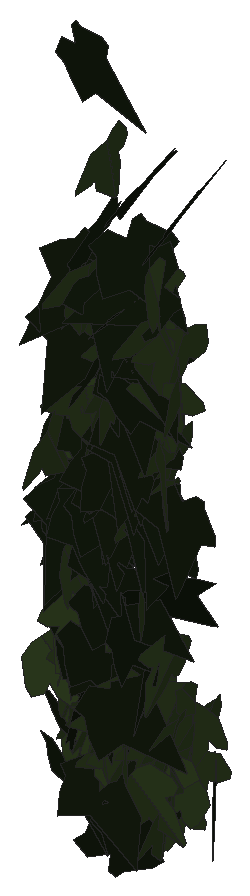
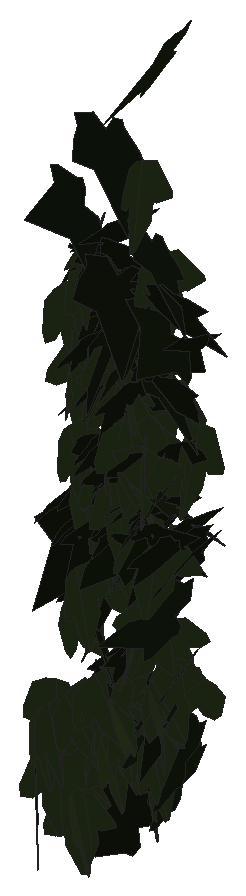
# SketchUp Ruby script. Lengths in inches.
U = 1.inch
M = Sketchup.active_model
def pt(a) = Geom::Point3d.new(a.map { |v| v * U })
def face(e, loops, mat)
  f = e.add_face(loops[0].map { |a| pt(a) })
  loops[1..].each { |l| e.add_face(l.map { |a| pt(a) }).erase! }
  f.material = f.back_material = mat if mat
  f
end
# faces: each face lists its corners as indices into pts; further lists are holes
def faces(e, pts, list, mat = nil) = list.each { |f| face(e, (f[0].is_a?(Array) ? f : [f]).map { |l| l.map { |i| pts[i] } }, mat) }
# xy, xz, yz: faces in a plane at the given z, y or x. An outline is a flat list of corners, or four numbers for a rectangle; further outlines are holes
def ring(l) = l.size == 4 ? [[l[0], l[1]], [l[2], l[1]], [l[2], l[3]], [l[0], l[3]]] : l.each_slice(2).to_a
def flat(e, list, mat, &to3) = list.each { |f| face(e, (f[0].is_a?(Array) ? f : [f]).map { |l| ring(l).map { |u, v| to3.(u, v) } }, mat) }
def xy(e, z, list, mat = nil) = flat(e, list, mat) { |x, y| [x, y, z] }
def xz(e, y, list, mat = nil) = flat(e, list, mat) { |x, z| [x, y, z] }
def yz(e, x, list, mat = nil) = flat(e, list, mat) { |y, z| [x, y, z] }
def lines(e, pts, list) = list.each { |a, b| e.add_line(pt(pts[a]), pt(pts[b])) }
# prism: a flat outline (further loops are holes) pulled along v
def prism(e, loops, v, mat = nil)
  f = face(e, loops, mat); d = Geom::Vector3d.new(v.map { |x| x * U })
  f.pushpull(f.normal.samedirection?(d) ? d.length : -d.length)
end
def box(e, o, s, mat = nil) = prism(e, [[o, [o[0] + s[0], o[1], o[2]], [o[0] + s[0], o[1] + s[1], o[2]], [o[0], o[1] + s[1], o[2]]]], [0, 0, s[2]], mat)
def at(x, y, z, deg = 0) = Geom::Transformation.translation(pt([x, y, z])) * Geom::Transformation.rotation(ORIGIN, Z_AXIS, deg.degrees)
def axes(o, x, y, z) = Geom::Transformation.new([*x, 0, *y, 0, *z, 0, *pt(o).to_a, 1])
def part(name) = M.definitions.add(name)
# library, detail: a bought-in or finely detailed component or shape, given as its bounding box
def library(name, o, s) = part(name).tap { |d| box(d.entities, o, s) }
def detail(e, o, s) = box(e.add_group.entities, o, s)
def put(e, d, t, mat = nil) = e.add_instance(d, t).tap { |i| i.material = mat if mat }
def group(e, t, mat = nil) = e.add_group.tap { |g| g.transformation = t; g.material = mat if mat }.entities
root = M.entities
M.materials.add("efeu1").color = [18, 25, 13]
M.materials.add("efeu2").color = [43, 57, 29]
c1 = part("ivyleaf_9")
p = [[1.54,2.16,1.25],[1.36,2.04,1.19],[-0.21,0.99,0.68],[-0.71,1.11,0.82],[-0.85,0.86,0.67],[-0.8,0.17,0.21],
  [-0.9,-0.01,0.1],[-0.67,-0.16,-0.02],[-0.08,-0.08,-0.05],[-0.03,-0.6,-0.4],[0.65,-0.88,-0.66],[0.83,-0.6,-0.49],
  [1.29,-0.42,-0.43],[1.8125,-0.07,-0.26],[1.21,0.44,0.15]]
faces(c1.entities,p,[[0,1,2,3,4,5,6,7,8,9,10,11,12,13,14]],"efeu1")
c2 = part("ivyleaf_10")
p = [[0,0.5,-0.03],[-0.0625,2.02,-0.43],[-0.19,2.01,-0.46],[-0.54,1.05,-0.29],[-0.52,0.625,-0.18],[-0.83,0.76,-0.28],
  [-1.16,0.64,-0.33],[-1.15,0.33,-0.24],[-0.77,-0.39,0.02],[-0.3,-0.51,0.16],[0.04,-0.48,0.23],[-0.02,2.01,-0.4375],
  [-0.06,2.01,-0.43],[0.04,-0.49,0.23],[0.67,-0.49,0.14],[1.38,0.36,-0.2],[1.375,0.51,-0.24],[0.81,0.65,-0.19],
  [0.62,0.59,-0.15],[0.6,1.09,-0.28],[0.5,1.23,-0.31]]
faces(c2.entities,p,[[0,1,2,3,4,5,6,7,8,9,10],[11,12,0,13,14,15,16,17,18,19,20]],"efeu2")
put(root,c1,axes([519.4,136.41,189.33],[0.62786,-0.42053,0.09806],[0.1674,0.07754,-0.73935],[0.39804,0.63072,0.15627]))
put(root,c2,axes([519.98,134.74,192.76],[0.04873,-0.68093,-0.48319],[0.02855,0.48508,-0.68073],[0.83446,0.02316,0.05151]))
put(root,c1,axes([519.65,136.01,190.9],[0.17877,-0.60551,-0.44438],[-0.02732,0.45125,-0.62586],[0.75058,0.16064,0.08305]))
put(root,c2,axes([519.98,136.06,187.02],[-0.04019,-0.69972,0.37768],[0.10675,-0.37948,-0.69171],[0.78794,0.01572,0.11298]))
put(root,c2,axes([520.09,136.15,185.5],[0.02126,-0.75748,0.0329],[-0.00474,-0.03305,-0.75775],[0.75818,0.02103,-0.00566]))
put(root,c1,axes([519.84,135.76,189.91],[-0.09217,-0.66346,0.40385],[-0.01785,-0.40476,-0.66905],[0.77651,-0.08806,0.03256]))
put(root,c1,axes([520.24,135.45,195.7],[0.19526,0.4822,0.58386],[-0.07597,0.61239,-0.48036],[-0.75342,0.06322,0.19976]))
put(root,c2,axes([519.59,135.28,187.0625],[0.53061,0.2169,0.52994],[0.49579,0.18745,-0.57313],[-0.28649,0.72612,-0.01034]))
put(root,c2,axes([520.15,136.03,190.54],[-0.6067,-0.44748,-0.06254],[0.0541,0.03201,-0.75384],[0.44858,-0.60907,0.00633]))
put(root,c1,axes([519.57,135.82,185.35],[0.53841,-0.59019,0.23254],[0.1518,-0.17626,-0.79886],[0.61592,0.55937,-0.00638]))
put(root,c1,axes([520.35,136.34,190.97],[-0.6514,-0.3842,0.08037],[-0.05254,-0.06898,-0.75556],[0.38898,-0.6527,0.03254]))
put(root,c2,axes([520.12,135.96,186.95],[0.28744,-0.67212,0.24553],[0.10655,-0.22145,-0.73093],[0.70758,0.30638,0.01032]))
put(root,c1,axes([520.51,135.22,186.4],[-0.1296,0.18302,-0.8633],[-0.7072,0.50041,0.21225],[0.52789,0.71532,0.0724]))
put(root,c1,axes([520.49,135.65,196.62],[-0.76491,-0.15378,0.03302],[-0.03296,-0.00358,-0.78021],[0.15379,-0.76562,-0.00298]))
put(root,c1,axes([519.79,136.01,187.22],[0.46827,-0.69757,-0.12739],[-0.04858,0.12074,-0.83974],[0.70744,0.47002,0.02666]))
put(root,c2,axes([520.1,136.32,188.6875],[-0.70161,0.1002,-0.25745],[0.22922,-0.18107,-0.69516],[-0.1542,-0.72509,0.13802]))
put(root,c2,axes([520.3,135.5625,188.23],[0.64412,0.32436,-0.21371],[-0.20684,-0.06387,-0.72035],[-0.32878,0.67563,0.0345]))
put(root,c1,axes([520.16,135.81,190.6],[-0.24349,-0.77579,0.29791],[-0.04142,-0.29871,-0.81175],[0.82999,-0.2425,0.04688]))
put(root,c1,axes([520.25,135.73,195.21],[-0.32979,-0.68595,0.20589],[-0.04139,-0.20803,-0.7594],[0.71499,-0.32844,0.05101]))
put(root,c1,axes([519.98,136.4,191.83],[0.35759,-0.6709,0.03227],[0.01369,-0.02927,-0.76025],[0.67154,0.35785,-0.00169]))
put(root,c2,axes([520.42,135.93,192.8],[0.2286,-0.6462,-0.38629],[-0.02349,0.39738,-0.67866],[0.75249,0.20872,0.09616]))
put(root,c1,axes([520.81,135.3,197.67],[-0.37796,0.6646,0.18343],[-0.08653,0.16181,-0.76455],[-0.684,-0.38771,-0.00465]))
put(root,c1,axes([520.84,135.58,191.73],[-0.71734,0.25796,-0.01039],[-0.06316,-0.20511,-0.73155],[-0.25032,-0.68747,0.21436]))
put(root,c1,axes([520.2,136.01,192.9],[-0.15486,-0.71167,-0.27805],[0.12148,0.25716,-0.72586],[0.75433,-0.18751,0.05981]))
put(root,c1,axes([520.84,135.32,194.71],[-0.51151,0.57612,0.00569],[-0.0038,0.00424,-0.77043],[-0.57614,-0.51152,0.00003]))
put(root,c1,axes([519.96,135.39,184.47],[0.43787,-0.63856,0.29211],[0.15808,-0.24577,-0.77422],[0.68417,0.46546,-0.00807]))
put(root,c2,axes([520.54,135.58,185.8],[0.29672,-0.6997,-0.07179],[-0.03319,0.0639,-0.76],[0.70259,0.29852,-0.00558]))
put(root,c2,axes([520.61,135.62,186.35],[0.51304,-0.43163,-0.3141],[-0.17742,0.27302,-0.66495],[0.50347,0.53604,0.08575]))
put(root,c2,axes([520.17,136.1,192.6875],[0.56352,0.40652,0.34786],[0.27327,0.21566,-0.69472],[-0.45999,0.62614,0.01343]))
put(root,c1,axes([520.16,135.89,194.82],[-0.27577,-0.37786,-0.6264],[0.57469,0.30231,-0.43537],[0.45264,-0.61404,0.17112]))
put(root,c2,axes([520.66,134.69,189.99],[-0.13696,0.64036,0.37512],[-0.2095,0.33258,-0.64423],[-0.71196,-0.22105,0.11741]))
put(root,c1,axes([520.16,136.125,185.95],[0.17917,-0.60388,0.43948],[0.20261,-0.3957,-0.62633],[0.71886,0.26204,0.067]))
put(root,c2,axes([520.75,136.17,193.22],[-0.45908,-0.60779,0.09787],[-0.00657,-0.11724,-0.75891],[0.61558,-0.45452,0.06489]))
put(root,c2,axes([520.6,135.9,188.55],[0.35102,-0.52158,-0.4512],[0.08319,0.53461,-0.55328],[0.68462,0.20246,0.29857]))
put(root,c2,axes([520.68,135.84,199.6],[0.02593,-0.73809,-0.27683],[0.06451,0.27803,-0.73526],[0.78565,0.00153,0.06951]))
put(root,c2,axes([520.76,135.07,196.86],[-0.14423,-0.79271,-0.04404],[0.00998,0.04295,-0.80573],[0.79387,-0.14456,0.00213]))
put(root,c2,axes([520.59,136.78,186.67],[0.36325,-0.59799,0.30121],[0.14821,-0.26237,-0.69962],[0.65296,0.39223,-0.00877]))
put(root,c2,axes([520.6875,135.68,191.68],[0.40284,-0.70378,0.09839],[0.03079,-0.09571,-0.81065],[0.70996,0.40348,-0.02067]))
put(root,c1,axes([520.4,136.375,194.78],[0.21017,-0.66144,-0.31804],[-0.04099,0.31973,-0.69204],[0.73278,0.20759,0.05251]))
put(root,c2,axes([520.78,135.13,193.83],[-0.7091,-0.36715,-0.06502],[0.0577,0.02998,-0.79851],[0.36837,-0.71145,-0.00009]))
put(root,c2,axes([520.78,135.5,184.5],[0.45996,-0.53802,-0.18395],[-0.06451,0.1857,-0.70443],[0.56493,0.45925,0.06933]))
put(root,c2,axes([520.36,135.32,185.7],[0.43547,-0.05792,0.65914],[0.64967,-0.11225,-0.43908],[0.12551,0.78199,-0.01421]))
put(root,c1,axes([520.58,135.03,202.44],[0.60057,-0.47896,-0.30462],[-0.14232,0.30225,-0.75583],[0.54949,0.60177,0.13718]))
put(root,c2,axes([521.03,136.11,191.62],[-0.30817,-0.70176,-0.06135],[0.02405,0.05644,-0.76644],[0.70402,-0.30911,-0.00067]))
put(root,c1,axes([520.73,135.34,190.98],[0.00331,-0.75327,-0.10452],[0.00542,0.10454,-0.75325],[0.76047,0.00254,0.00582]))
put(root,c2,axes([521.02,135.62,194.07],[0.23431,-0.72389,0.15536],[0.03955,-0.15048,-0.76082],[0.73932,0.23747,-0.00854]))
put(root,c2,axes([520.53,135.98,193.67],[0.56017,-0.01498,0.54702],[0.54381,0.10249,-0.55408],[-0.061,0.77621,0.08372]))
put(root,c1,axes([520.63,136.2,190.86],[0.72569,-0.23795,-0.02613],[-0.02865,-0.00352,-0.76361],[0.23766,0.72615,-0.01227]))
put(root,c1,axes([521.29,135.93,196.92],[-0.04492,0.78645,0.02013],[-0.00595,0.01982,-0.78771],[-0.78668,-0.04506,0.00481]))
put(root,c1,axes([520.83,135.42,187.8],[0.18152,-0.58271,-0.50064],[-0.12002,0.48659,-0.60988],[0.7588,0.21636,0.02329]))
put(root,c1,axes([521,135.99,190.78],[-0.23052,-0.72721,0.07545],[-0.03857,-0.0669,-0.7627],[0.7301,-0.23314,-0.01647]))
put(root,c2,axes([521.23,135.86,194.88],[-0.55356,-0.56218,-0.01701],[0.01551,0.0086,-0.78895],[0.56222,-0.55375,0.00502]))
put(root,c1,axes([520.86,135.32,191.36],[0.32309,-0.53201,-0.48751],[-0.13922,0.47815,-0.61406],[0.70803,0.33678,0.10171]))
put(root,c1,axes([521,135.81,192.03],[-0.17758,-0.73878,-0.07039],[0.00817,0.07043,-0.75977],[0.74208,-0.17756,-0.00848]))
put(root,c2,axes([521.38,135.58,195.34],[-0.74846,-0.15183,0.18018],[-0.17887,-0.02442,-0.76362],[0.15336,-0.76946,-0.01132]))
put(root,c1,axes([520.97,135.79,195.55],[0.63397,-0.27567,-0.37961],[-0.32663,0.19873,-0.68981],[0.33677,0.71171,0.04558]))
put(root,c2,axes([521.15,135.93,193.99],[-0.31921,-0.69501,-0.09899],[0.15218,0.03765,-0.75508],[0.68533,-0.33208,0.12156]))
put(root,c1,axes([520.86,135,188.1],[0.35936,-0.59923,-0.3386],[-0.1068,0.3288,-0.69523],[0.67994,0.36835,0.06975]))
put(root,c2,axes([521.51,135.81,186.14],[-0.18237,-0.08826,-0.71353],[-0.48298,-0.53026,0.18903],[-0.53259,0.51109,0.0729]))
put(root,c1,axes([521.05,135.89,191.37],[-0.00932,-0.77797,0.06994],[0.0057,-0.07001,-0.77799],[0.78108,-0.00877,0.00651]))
put(root,c1,axes([521.59,135.21,185.91],[-0.62481,0.41863,-0.27449],[-0.23116,0.14811,0.75207],[0.44403,0.66618,0.00529]))
put(root,c2,axes([521.13,135.9,194.42],[0.71282,0.32212,0.08483],[0.07357,0.04316,-0.78218],[-0.32488,0.71655,0.00898]))
put(root,c2,axes([521.42,135.43,185.35],[-0.21378,-0.70046,0.08652],[-0.0136,-0.0863,-0.73226],[0.70565,-0.21388,0.01209]))
put(root,c1,axes([520.98,135.4375,189.96],[0.16661,-0.75373,0.15222],[0.04137,-0.14674,-0.77188],[0.76783,0.17145,0.00856]))
put(root,c2,axes([521.4,135.34,185.63],[0.55029,-0.35981,-0.33528],[-0.13037,0.37841,-0.62008],[0.47421,0.52157,0.21859]))
put(root,c2,axes([521.37,135.0625,194.22],[0.22658,-0.50207,-0.54988],[0.01335,0.57743,-0.52171],[0.74449,0.14245,0.17671]))
put(root,c2,axes([520.79,135.47,185.35],[0.14682,-0.1247,-0.76849],[0.77854,0.02002,0.14549],[-0.00348,-0.78214,0.12625]))
put(root,c2,axes([521.53,136.2,186.64],[-0.38994,-0.58021,0.28819],[-0.02332,-0.32357,-0.68301],[0.64742,-0.36112,0.14897]))
put(root,c2,axes([521.57,135.37,186.25],[-0.41024,-0.69039,0.14792],[-0.06359,-0.13425,-0.80296],[0.70319,-0.41491,0.01368]))
put(root,c2,axes([521.47,135.78,192.23],[0.17972,-0.72252,-0.20188],[-0.00182,0.20717,-0.74308],[0.75019,0.1736,0.04656]))
put(root,c2,axes([521.49,135.95,185.07],[0.14745,-0.72736,0.01988],[0.00361,-0.01956,-0.74215],[0.72762,0.14749,-0.00035]))
put(root,c2,axes([521.48,135.59,185.25],[-0.06257,-0.70016,0.30085],[0.06637,-0.30572,-0.69769],[0.75916,-0.03098,0.08579]))
put(root,c1,axes([521.3125,135.53,196.56],[-0.16673,-0.76447,-0.01786],[0.00277,0.01767,-0.78244],[0.76467,-0.16675,-0.00106]))
put(root,c2,axes([521.55,137.03,183.95],[0.27725,-0.66783,-0.04679],[-0.01529,0.04431,-0.72308],[0.66929,0.27766,0.00286]))
put(root,c1,axes([521.27,135.09,184.83],[-0.14683,-0.59699,-0.45984],[0.16555,0.43149,-0.61304],[0.73514,-0.21641,0.04621]))
put(root,c1,axes([521.87,135.17,196.46],[-0.03679,0.77537,0.07741],[-0.10273,0.072,-0.76994],[-0.77242,-0.0465,0.09871]))
put(root,c2,axes([521.64,135.51,186.75],[0.00618,-0.56856,0.52102],[0.00671,-0.52098,-0.5686],[0.77115,0.00909,0.00078]))
put(root,c1,axes([521.69,135.71,195.88],[0.52731,0.07387,-0.59041],[-0.59406,0.10985,-0.51683],[0.03356,0.78394,0.12805]))
put(root,c1,axes([521.39,136.01,192.86],[-0.02275,-0.7828,0.01386],[-0.01219,-0.01351,-0.78304],[0.78283,-0.02296,-0.01179]))
put(root,c1,axes([521.38,135.51,192.23],[0.05825,-0.68428,-0.36084],[-0.03084,0.35952,-0.68675],[0.77298,0.06591,-0.00021]))
put(root,c2,axes([521.72,136.69,189.4375],[0.03823,-0.7428,-0.0518],[-0.01063,0.05132,-0.74374],[0.74453,0.03887,-0.00796]))
put(root,c1,axes([521.375,136.07,190.87],[0.10045,-0.61787,-0.45979],[0.0235,0.46593,-0.62098],[0.76982,0.0664,0.07895]))
put(root,c1,axes([521.42,135.95,193.13],[0.04118,-0.78587,-0.00932],[-0.0003,0.00932,-0.78695],[0.78593,0.04118,0.00019]))
put(root,c1,axes([521.58,136,193],[-0.27906,-0.73042,0.00033],[-0.00467,0.00144,-0.78189],[0.7304,-0.27905,-0.00487]))
put(root,c2,axes([521.86,135.57,189.25],[-0.35648,-0.5293,0.39902],[-0.08054,-0.41512,-0.62261],[0.65794,-0.3376,0.13998]))
put(root,c2,axes([521.91,136.61,183.68],[-0.66975,-0.13316,0.18494],[-0.17162,-0.08305,-0.68128],[0.14994,-0.68983,0.04633]))
put(root,c2,axes([521.83,135.73,190.5625],[0.53519,-0.45649,-0.30923],[-0.12529,0.31899,-0.68774],[0.53695,0.52943,0.14774]))
put(root,c1,axes([521.4,135.2,182.87],[0.01776,-0.08125,0.79188],[0.74794,0.27285,0.01122],[-0.2725,0.7436,0.08241]))
put(root,c1,axes([521.58,135.74,194.5],[0.1029,-0.7898,0.02099],[0.00251,-0.02084,-0.79648],[0.79008,0.10293,-0.00021]))
put(root,c2,axes([521.95,136.66,186.23],[-0.0795,-0.67236,0.28448],[0.01993,-0.28805,-0.67524],[0.72979,-0.06537,0.04943]))
put(root,c2,axes([521.95,135.66,191.52],[-0.0381,-0.71019,-0.293],[0.04411,0.29085,-0.71073],[0.76699,-0.05201,0.02632]))
put(root,c1,axes([521.65,135.02,194.59],[0.61701,-0.35369,-0.29662],[-0.11361,0.36357,-0.66985],[0.44741,0.58009,0.23897]))
put(root,c2,axes([522.1,135.9,185.58],[-0.21393,-0.69356,0.05873],[-0.01569,-0.05662,-0.72581],[0.69587,-0.2145,0.00168]))
put(root,c1,axes([522.53,135.375,197.07],[-0.72532,0.01635,0.30216],[-0.3021,-0.08465,-0.72058],[0.01756,-0.78117,0.08441]))
put(root,c1,axes([521.71,134.8,187.05],[0.34969,-0.51406,-0.57933],[-0.08296,0.60713,-0.5888],[0.77007,0.29884,0.19964]))
put(root,c1,axes([522.04,134.75,189.01],[0.34391,-0.28914,-0.66596],[-0.48239,0.45971,-0.44871],[0.54259,0.59198,0.02318]))
put(root,c1,axes([521.68,135.39,197.87],[0.25714,-0.63486,-0.4056],[0.04837,0.44161,-0.66055],[0.75181,0.18873,0.18122]))
put(root,c1,axes([522.4,134.96,199.76],[-0.24166,0.76746,0.00714],[-0.00165,0.00697,-0.80461],[-0.76749,-0.24166,-0.00052]))
put(root,c2,axes([522.08,136.15,191.44],[0.14622,-0.70765,0.31109],[0.11362,-0.29349,-0.72102],[0.76461,0.17894,0.04765]))
put(root,c1,axes([521.68,134.77,189.55],[-0.05433,-0.1559,-0.79226],[0.35287,0.70962,-0.16383],[0.72626,-0.35645,0.02034]))
put(root,c1,axes([522.05,135.73,187.8],[-0.50433,0.15283,-0.57285],[0.55102,-0.15676,-0.52693],[-0.21883,-0.74695,-0.00662]))
put(root,c2,axes([522.19,136.3125,192.67],[0.03726,-0.76654,-0.001],[0,0.001,-0.76744],[0.76654,0.03726,0.00005]))
put(root,c2,axes([522.29,136.78,184.67],[-0.58262,-0.45077,0.07123],[-0.06645,-0.0305,-0.73646],[0.4515,-0.58617,-0.01646]))
put(root,c2,axes([522.28,135,189.71],[0.33104,-0.35753,-0.58055],[-0.11603,0.60641,-0.43961],[0.67187,0.28088,0.21013]))
put(root,c1,axes([521.875,135.875,195.34],[0.1583,-0.75586,-0.16787],[-0.00334,0.17067,-0.77164],[0.77427,0.15527,0.03099]))
put(root,c1,axes([522.03,135.81,191.61],[-0.11345,-0.7558,0.01866],[-0.00227,-0.01852,-0.76427],[0.75603,-0.11347,0.00051]))
put(root,c2,axes([522.69,136.18,184.46],[-0.43132,0.07761,0.56223],[-0.53593,-0.28817,-0.37136],[0.18684,-0.64739,0.23271]))
put(root,c2,axes([522.4,135.52,194.29],[-0.67992,-0.37141,-0.06905],[0.06062,0.03305,-0.77475],[0.37288,-0.68262,0.00005]))
put(root,c1,axes([522.46,135.74,198.25],[-0.34667,0.56148,-0.44715],[-0.22481,0.38665,0.65981],[0.68166,0.41307,-0.00981]))
put(root,c2,axes([522.4375,135.9,185.86],[0.1228,-0.72769,0.01937],[0.00162,-0.01937,-0.73798],[0.72795,0.1228,-0.00162]))
put(root,c2,axes([521.93,136.28,184.67],[-0.20507,-0.00416,0.72934],[0.66836,-0.30435,0.18619],[0.29196,0.6938,0.08605]))
put(root,c2,axes([522.48,136.71,185.78],[-0.02259,-0.74387,0.01041],[0.00262,-0.01049,-0.74421],[0.74394,-0.02255,0.00294]))
put(root,c2,axes([522.52,137.01,185.75],[0.09195,-0.71424,-0.05387],[0.00422,0.05485,-0.72005],[0.71626,0.09137,0.01115]))
put(root,c2,axes([522.54,135.45,184.05],[0.17043,-0.69045,-0.23697],[-0.02242,0.23827,-0.71038],[0.72964,0.1686,0.03352]))
put(root,c2,axes([522.7,136.44,186.17],[-0.71039,0.08947,0.19301],[-0.19825,-0.03442,-0.71374],[-0.07715,-0.73534,0.05689]))
put(root,c1,axes([522.33,136.06,190.74],[-0.05742,-0.66271,0.37873],[-0.02391,-0.37806,-0.66515],[0.76292,-0.06173,0.00766]))
put(root,c2,axes([522.63,135.18,196.21],[-0.13602,-0.80427,-0.03819],[-0.00072,0.03885,-0.81566],[0.80518,-0.13583,-0.00718]))
put(root,c2,axes([522.19,135.84,192.46],[0.27032,-0.38703,0.60995],[0.54746,-0.31514,-0.44259],[0.4713,0.58805,0.16426]))
put(root,c2,axes([522.65,135.7,188.03],[0.03383,-0.63617,0.40051],[0.09173,-0.39443,-0.63425],[0.74613,0.07733,0.05982]))
put(root,c2,axes([522.26,135.19,184.73],[-0.44683,0.0973,-0.60337],[0.55178,-0.25716,-0.4501],[-0.26279,-0.70539,0.08087]))
put(root,c2,axes([522.625,135.14,197.21],[-0.22482,0.76053,0.0821],[-0.02651,0.07777,-0.79305],[-0.76449,-0.22635,0.00336]))
put(root,c1,axes([523.0625,136.59,184.17],[0.07919,-0.01037,-0.77865],[-0.74257,0.23468,-0.07864],[0.23449,0.74665,0.01391]))
put(root,c2,axes([522.85,135.68,195.73],[-0.21555,-0.7521,0.12961],[-0.02693,-0.1271,-0.78232],[0.76271,-0.21704,0.00901]))
put(root,c2,axes([522.78,135.63,194.64],[0.321,-0.63192,-0.37242],[-0.01445,0.40099,-0.69286],[0.73336,0.2845,0.14936]))
put(root,c1,axes([522.5,136.16,191.34],[0.01506,-0.74074,0.19515],[0.0429,-0.19407,-0.73993],[0.76481,0.02547,0.03766]))
put(root,c1,axes([522.6,135.04,189.75],[0.56592,0.49019,0.12833],[0.10203,0.0782,-0.74866],[-0.49633,0.57499,-0.00758]))
